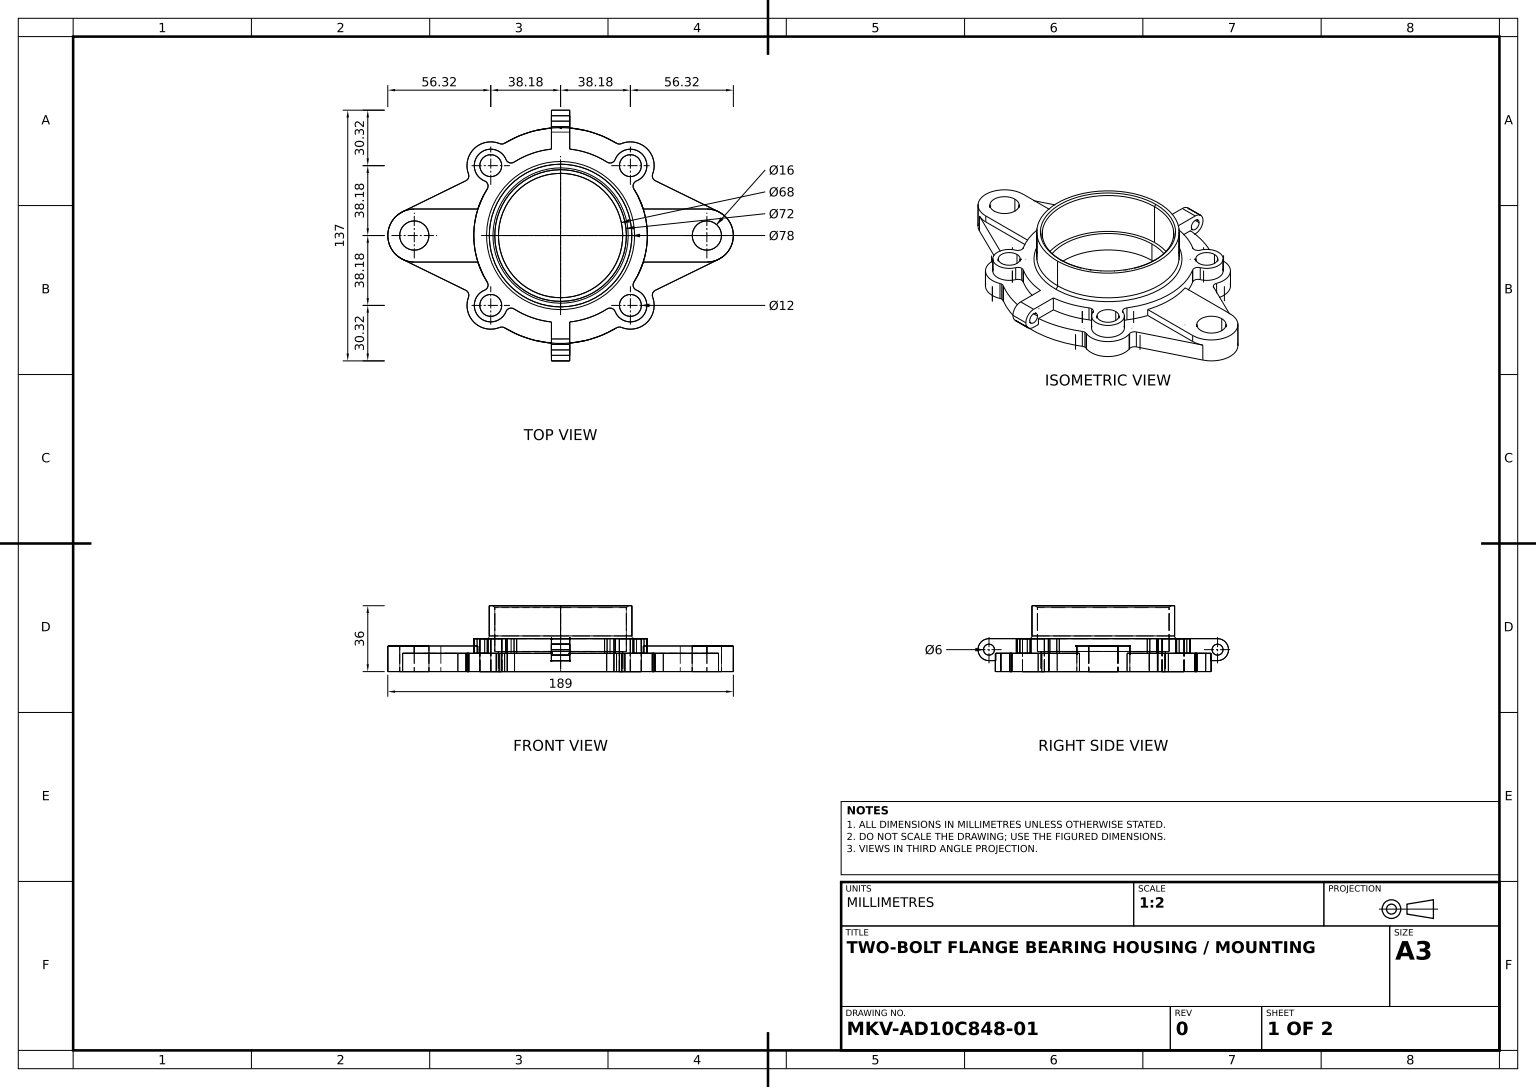
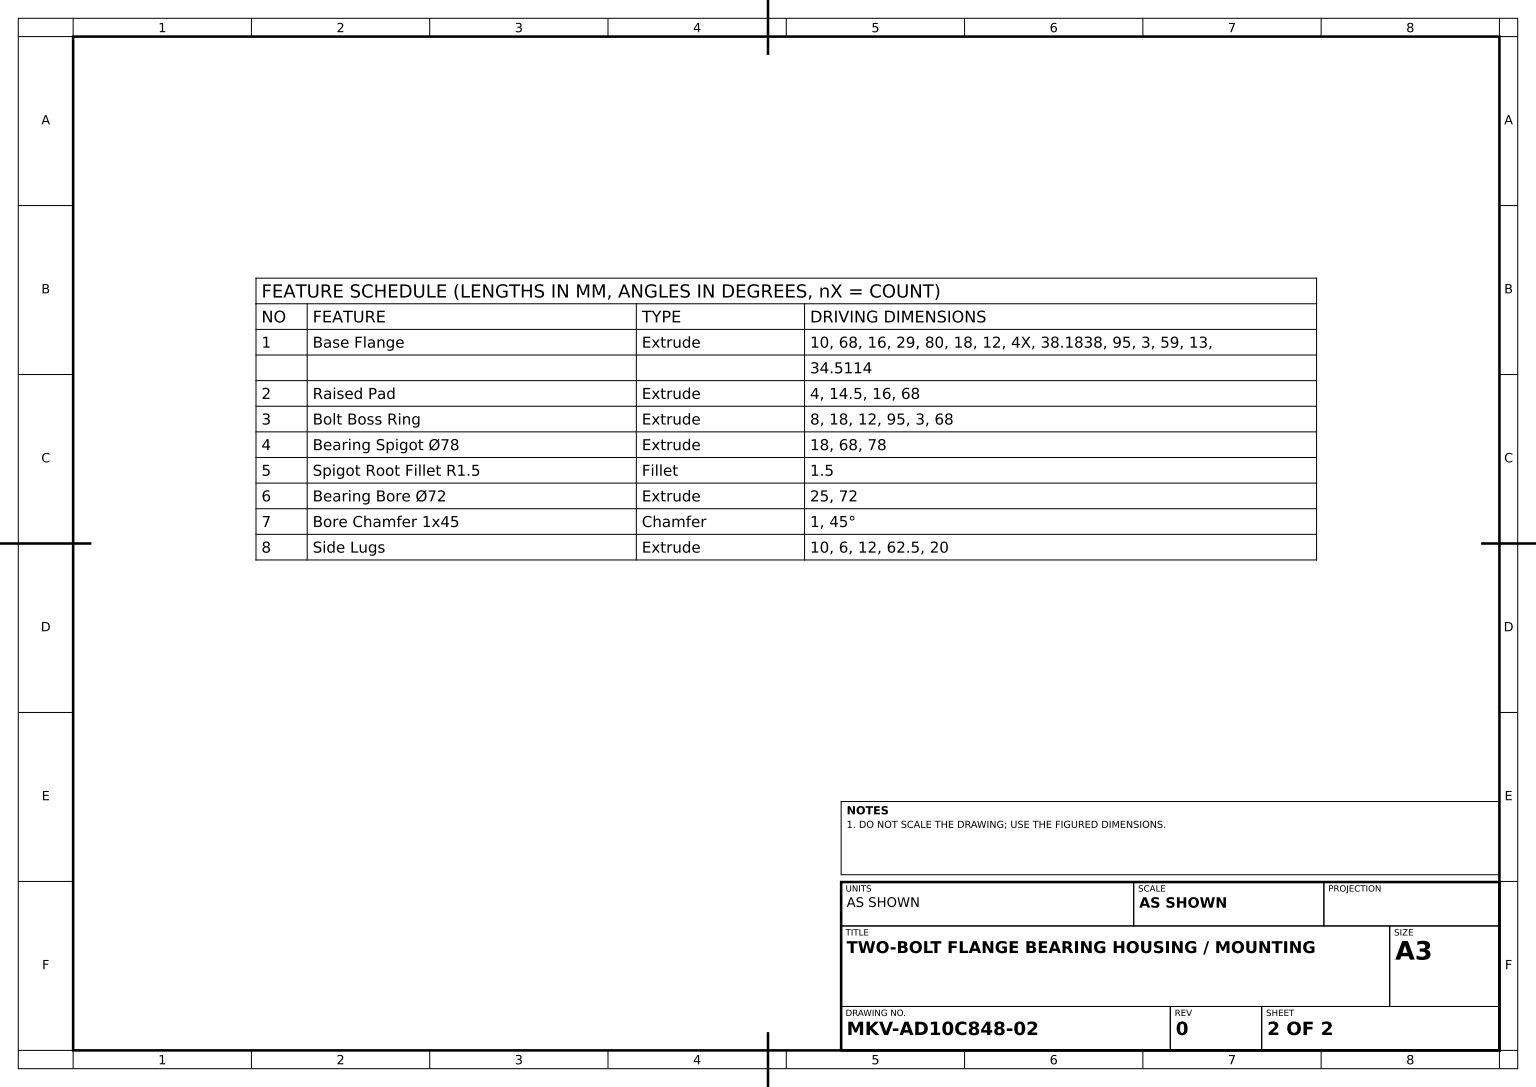
solid
v1 (5,10,47.236109)
v2 (25.438297,10,40.114125)
e1 v1 v2 CIRCLE(AX(P(0,10,0),D(0,1,0),D(0,0,1)),47.5)
v3 (25.438297,18,40.114125)
e2 v3 v2 LINE
v4 (5,18,47.236109)
e3 v4 v3 CIRCLE(AX(P(0,18,0),D(0,1,0),D(0,0,1)),47.5)
e4 v4 v1 LINE
face CYL(AX(P(0,18,0),D(0,-1,0),D(0,0,-1)),47.5) [e1 -e2 -e3 e4]
v5 (-30.604247,0,-50.441848)
v6 (-33.289778,0,-50.22739)
e5 v5 v6 CIRCLE(AX(P(-32.160396,0,-53.006688),D(0,-1,0),D(0,0,1)),3)
v7 (-33.289778,10,-50.22739)
e6 v7 v6 LINE
v8 (-30.604247,10,-50.441848)
e7 v8 v7 CIRCLE(AX(P(-32.160396,10,-53.006688),D(0,-1,0),D(0,0,1)),3)
e8 v8 v5 LINE
face CYL(AX(P(-32.160396,10,-53.006688),D(0,-1,0),D(0,0,-1)),3) rev [e5 -e6 -e7 e8]
v9 (38.183766,18,44.183766)
v10 (38.183766,18,32.183766)
e9 v9 v10 CIRCLE(AX(P(38.183766,18,38.183766),D(0,1,0),D(0,0,1)),6)
v11 (38.183766,0,32.183766)
e10 v10 v11 LINE
v12 (38.183766,0,44.183766)
e11 v12 v11 CIRCLE(AX(P(38.183766,0,38.183766),D(0,1,0),D(0,0,1)),6)
e12 v9 v12 LINE
face CYL(AX(P(38.183766,10,38.183766),D(0,-1,0),D(0,0,-1)),6) rev [e9 e10 -e11 -e12]
v13 (80,14,8)
v14 (80,0,8)
e13 v13 v14 LINE
v15 (80,14,-8)
e14 v13 v15 CIRCLE(AX(P(80,14,0),D(0,1,0),D(0,0,1)),8)
v16 (80,0,-8)
e15 v15 v16 LINE
e16 v14 v16 CIRCLE(AX(P(80,0,0),D(0,1,0),D(0,0,1)),8)
face CYL(AX(P(80,10,0),D(0,-1,0),D(0,0,-1)),8) rev [-e13 e14 e15 -e16]
v17 (27.044926,10,39.647649)
e17 v2 v17 CIRCLE(AX(P(27.044926,10,42.647649),D(0,-1,0),D(0,0,1)),3)
v18 (27.044926,18,39.647649)
e18 v18 v17 LINE
e19 v3 v18 CIRCLE(AX(P(27.044926,18,42.647649),D(0,-1,0),D(0,0,1)),3)
face CYL(AX(P(27.044926,18,42.647649),D(0,-1,0),D(0,0,-1)),3) rev [e17 -e18 -e19 e2]
v19 (29.829636,18,41.531678)
v20 (29.829636,10,41.531678)
e20 v19 v20 LINE
e21 v18 v19 CIRCLE(AX(P(27.044926,18,42.647649),D(0,-1,0),D(0,0,1)),3)
e22 v17 v20 CIRCLE(AX(P(27.044926,10,42.647649),D(0,-1,0),D(0,0,1)),3)
face CYL(AX(P(27.044926,18,42.647649),D(0,-1,0),D(0,0,-1)),3) rev [-e20 -e21 e18 e22]
v21 (-41.531678,18,-29.829636)
v22 (-41.531678,10,-29.829636)
e23 v21 v22 LINE
v23 (-38.183766,18,-47.183766)
e24 v23 v21 CIRCLE(AX(P(-38.183766,18,-38.183766),D(0,1,0),D(0,0,1)),9)
v24 (-38.183766,10,-47.183766)
e25 v23 v24 LINE
e26 v24 v22 CIRCLE(AX(P(-38.183766,10,-38.183766),D(0,1,0),D(0,0,1)),9)
face CYL(AX(P(-38.183766,18,-38.183766),D(0,-1,0),D(0,0,-1)),9) [-e23 -e24 e25 e26]
v25 (5,6,-62.5)
v26 (-5,6,-62.5)
e27 v25 v26 LINE
v27 (5,6,-58.787754)
e28 v27 v25 LINE
v28 (0,6,-59)
e29 v27 v28 CIRCLE(AX(P(0,6,0),D(0,1,0),D(0,0,1)),59)
v29 (-5,6,-58.787754)
e30 v28 v29 CIRCLE(AX(P(0,6,0),D(0,1,0),D(0,0,1)),59)
e31 v29 v26 LINE
face PLANE(AX(P(5,6,-42.5),D(0,1,0),D(0,0,1))) rev [-e27 -e28 e29 e30 e31]
v30 (32.160396,0,50.006688)
v31 (30.604247,0,50.441848)
e32 v30 v31 CIRCLE(AX(P(32.160396,0,53.006688),D(0,1,0),D(0,0,1)),3)
v32 (32.160396,10,50.006688)
e33 v32 v30 LINE
v33 (30.604247,10,50.441848)
e34 v32 v33 CIRCLE(AX(P(32.160396,10,53.006688),D(0,1,0),D(0,0,1)),3)
e35 v33 v31 LINE
face CYL(AX(P(32.160396,10,53.006688),D(0,-1,0),D(0,0,-1)),3) rev [-e32 -e33 e34 e35]
v34 (-50.367829,10,-33.650707)
v35 (-50.367829,0,-33.650707)
e36 v34 v35 LINE
v36 (-51.861087,0,-29.909864)
e37 v36 v35 CIRCLE(AX(P(-53.179535,0,-32.604617),D(0,1,0),D(0,0,1)),3)
v37 (-51.861087,10,-29.909864)
e38 v37 v36 LINE
e39 v37 v34 CIRCLE(AX(P(-53.179535,10,-32.604617),D(0,1,0),D(0,0,1)),3)
face CYL(AX(P(-53.179535,10,-32.604617),D(0,-1,0),D(0,0,-1)),3) rev [e36 -e37 -e38 e39]
v38 (-86.3725,10,-13.02464)
v39 (-86.3725,0,-13.02464)
e40 v38 v39 LINE
e41 v38 v37 LINE
e42 v39 v36 LINE
face PLANE(AX(P(-21.824105,10,-44.605905),D(-0.439482725,0,-0.898251042),D(-0.898251042,0,0.439482725))) [-e40 e41 e38 -e42]
v40 (0,11,-34)
v41 (0,11,34)
e43 v40 v41 CIRCLE(AX(P(0,11,0),D(0,1,0),D(0,0,1)),34)
v42 (0,0,34)
e44 v41 v42 LINE
v43 (0,0,-34)
e45 v43 v42 CIRCLE(AX(P(0,0,0),D(0,1,0),D(0,0,1)),34)
e46 v40 v43 LINE
face CYL(AX(P(0,10,0),D(0,-1,0),D(0,0,-1)),34) rev [e43 e44 -e45 -e46]
v44 (45.232732,14,-14.5)
v45 (45.232732,14,14.5)
e47 v44 v45 CIRCLE(AX(P(0,14,0),D(0,-1,0),D(0,0,1)),47.5)
v46 (45.232732,10,-14.5)
e48 v44 v46 LINE
v47 (40.114125,10,-25.438297)
e49 v46 v47 CIRCLE(AX(P(0,10,0),D(0,1,0),D(0,0,1)),47.5)
v48 (40.114125,18,-25.438297)
e50 v48 v47 LINE
v49 (40.114125,18,25.438297)
e51 v49 v48 CIRCLE(AX(P(0,18,0),D(0,1,0),D(0,0,1)),47.5)
v50 (40.114125,10,25.438297)
e52 v49 v50 LINE
v51 (45.232732,10,14.5)
e53 v50 v51 CIRCLE(AX(P(0,10,0),D(0,1,0),D(0,0,1)),47.5)
e54 v51 v45 LINE
face CYL(AX(P(0,18,0),D(0,-1,0),D(0,0,-1)),47.5) [-e47 e48 e49 -e50 -e51 e52 e53 e54]
v52 (38.183766,10,-51.183766)
v53 (33.289778,10,-50.22739)
e55 v52 v53 CIRCLE(AX(P(38.183766,10,-38.183766),D(0,1,0),D(0,0,1)),13)
v54 (38.183766,0,-51.183766)
e56 v52 v54 LINE
v55 (33.289778,0,-50.22739)
e57 v54 v55 CIRCLE(AX(P(38.183766,0,-38.183766),D(0,1,0),D(0,0,1)),13)
e58 v53 v55 LINE
face CYL(AX(P(38.183766,10,-38.183766),D(0,-1,0),D(0,0,-1)),13) [-e55 e56 e57 -e58]
v56 (30.604247,0,-50.441848)
e59 v55 v56 CIRCLE(AX(P(32.160396,0,-53.006688),D(0,-1,0),D(0,0,1)),3)
v57 (30.604247,10,-50.441848)
e60 v57 v56 LINE
e61 v53 v57 CIRCLE(AX(P(32.160396,10,-53.006688),D(0,-1,0),D(0,0,1)),3)
face CYL(AX(P(32.160396,10,-53.006688),D(0,-1,0),D(0,0,-1)),3) rev [e59 -e60 -e61 e58]
v58 (-80,14,14.5)
v59 (-80,10,14.5)
e62 v58 v59 LINE
v60 (-80,14,-14.5)
e63 v60 v58 CIRCLE(AX(P(-80,14,0),D(0,1,0),D(0,0,1)),14.5)
v61 (-80,10,-14.5)
e64 v60 v61 LINE
e65 v61 v38 CIRCLE(AX(P(-80,10,0),D(0,1,0),D(0,0,1)),14.5)
v62 (-86.3725,0,13.02464)
e66 v39 v62 CIRCLE(AX(P(-80,0,0),D(0,1,0),D(0,0,1)),14.5)
v63 (-86.3725,10,13.02464)
e67 v63 v62 LINE
e68 v59 v63 CIRCLE(AX(P(-80,10,0),D(0,-1,0),D(0,0,1)),14.5)
face CYL(AX(P(-80,10,0),D(0,-1,0),D(0,0,-1)),14.5) [-e62 -e63 e64 e65 e40 e66 -e67 -e68]
v64 (50.367829,10,33.650707)
v65 (50.367829,0,33.650707)
e69 v64 v65 LINE
v66 (51.861087,0,29.909864)
e70 v65 v66 CIRCLE(AX(P(53.179535,0,32.604617),D(0,-1,0),D(0,0,1)),3)
v67 (51.861087,10,29.909864)
e71 v67 v66 LINE
e72 v64 v67 CIRCLE(AX(P(53.179535,10,32.604617),D(0,-1,0),D(0,0,1)),3)
face CYL(AX(P(53.179535,10,32.604617),D(0,-1,0),D(0,0,-1)),3) rev [e69 e70 -e71 -e72]
v68 (-80,14,-8)
v69 (-80,14,8)
e73 v68 v69 CIRCLE(AX(P(-80,14,0),D(0,1,0),D(0,0,1)),8)
v70 (-80,0,8)
e74 v69 v70 LINE
v71 (-80,0,-8)
e75 v71 v70 CIRCLE(AX(P(-80,0,0),D(0,1,0),D(0,0,1)),8)
e76 v68 v71 LINE
face CYL(AX(P(-80,10,0),D(0,-1,0),D(0,0,-1)),8) rev [e73 e74 -e75 -e76]
v72 (-5,6,58.787754)
v73 (5,6,58.787754)
e77 v72 v73 CIRCLE(AX(P(0,6,0),D(0,1,0),D(0,0,1)),59)
v74 (5,6,62.5)
e78 v74 v73 LINE
v75 (-5,6,62.5)
e79 v74 v75 LINE
e80 v75 v72 LINE
face PLANE(AX(P(5,6,42.5),D(0,1,0),D(0,0,1))) rev [e77 -e78 e79 e80]
v76 (0,11,36)
v77 (0,35,36)
e81 v76 v77 LINE
v78 (0,35,-36)
e82 v77 v78 CIRCLE(AX(P(0,35,0),D(0,1,0),D(0,0,1)),36)
v79 (0,11,-36)
e83 v79 v78 LINE
e84 v76 v79 CIRCLE(AX(P(0,11,0),D(0,1,0),D(0,0,1)),36)
face CYL(AX(P(0,11,0),D(0,1,0),D(0,0,1)),36) rev [e81 e82 -e83 -e84]
v80 (80,10,14.5)
e85 v51 v80 LINE
v81 (80,14,14.5)
e86 v81 v80 LINE
e87 v45 v81 LINE
face PLANE(AX(P(80,14,14.5),D(0,0,-1),D(-1,0,0))) rev [e85 -e86 -e87 -e54]
v82 (-45.232732,14,-14.5)
e88 v82 v60 LINE
v83 (-45.232732,10,-14.5)
e89 v83 v82 LINE
e90 v83 v61 LINE
face PLANE(AX(P(-80,14,-14.5),D(0,0,1),D(1,0,0))) rev [-e64 -e88 -e89 e90]
v84 (-40.114125,10,25.438297)
v85 (-41.531678,10,29.829636)
e91 v84 v85 CIRCLE(AX(P(-42.647649,10,27.044926),D(0,-1,0),D(0,0,1)),3)
v86 (-45.232732,10,14.5)
e92 v86 v84 CIRCLE(AX(P(0,10,0),D(0,1,0),D(0,0,1)),47.5)
e93 v59 v86 LINE
v87 (-51.861087,10,29.909864)
e94 v63 v87 LINE
v88 (-50.367829,10,33.650707)
e95 v87 v88 CIRCLE(AX(P(-53.179535,10,32.604617),D(0,-1,0),D(0,0,1)),3)
v89 (-33.289778,10,50.22739)
e96 v88 v89 CIRCLE(AX(P(-38.183766,10,38.183766),D(0,1,0),D(0,0,1)),13)
v90 (-32.160396,10,50.006688)
e97 v90 v89 CIRCLE(AX(P(-32.160396,10,53.006688),D(0,1,0),D(0,0,1)),3)
v91 (-30.604247,10,50.441848)
e98 v91 v90 CIRCLE(AX(P(-32.160396,10,53.006688),D(0,1,0),D(0,0,1)),3)
v92 (-5,10,58.787754)
e99 v91 v92 CIRCLE(AX(P(0,10,0),D(0,1,0),D(0,0,1)),59)
v93 (-5,10,47.236109)
e100 v92 v93 LINE
v94 (-25.438297,10,40.114125)
e101 v94 v93 CIRCLE(AX(P(0,10,0),D(0,1,0),D(0,0,1)),47.5)
v95 (-27.044926,10,39.647649)
e102 v95 v94 CIRCLE(AX(P(-27.044926,10,42.647649),D(0,-1,0),D(0,0,-1)),3)
v96 (-29.829636,10,41.531678)
e103 v96 v95 CIRCLE(AX(P(-27.044926,10,42.647649),D(0,-1,0),D(0,0,-1)),3)
e104 v85 v96 CIRCLE(AX(P(-38.183766,10,38.183766),D(0,1,0),D(0,0,1)),9)
face PLANE(AX(P(0,10,0),D(0,1,0),D(0,0,1))) [-e91 -e92 -e93 e68 e94 e95 e96 -e97 -e98 e99 e100 -e101 -e102 -e103 -e104]
v97 (-25.438297,10,-40.114125)
v98 (-29.829636,10,-41.531678)
e105 v97 v98 CIRCLE(AX(P(-27.044926,10,-42.647649),D(0,-1,0),D(0,0,1)),3)
v99 (-29.829636,18,-41.531678)
e106 v99 v98 LINE
v100 (-25.438297,18,-40.114125)
e107 v100 v99 CIRCLE(AX(P(-27.044926,18,-42.647649),D(0,-1,0),D(0,0,1)),3)
e108 v100 v97 LINE
face CYL(AX(P(-27.044926,18,-42.647649),D(0,-1,0),D(0,0,-1)),3) rev [e105 -e106 -e107 e108]
v101 (25.438297,18,-40.114125)
v102 (25.438297,10,-40.114125)
e109 v101 v102 LINE
v103 (5,10,-47.236109)
e110 v102 v103 CIRCLE(AX(P(0,10,0),D(0,1,0),D(0,0,1)),47.5)
v104 (5,18,-47.236109)
e111 v103 v104 LINE
e112 v101 v104 CIRCLE(AX(P(0,18,0),D(0,1,0),D(0,0,1)),47.5)
face CYL(AX(P(0,18,0),D(0,-1,0),D(0,0,-1)),47.5) [e109 e110 e111 -e112]
v105 (51.861087,10,-29.909864)
v106 (50.367829,10,-33.650707)
e113 v105 v106 CIRCLE(AX(P(53.179535,10,-32.604617),D(0,-1,0),D(0,0,1)),3)
v107 (51.861087,0,-29.909864)
e114 v105 v107 LINE
v108 (50.367829,0,-33.650707)
e115 v107 v108 CIRCLE(AX(P(53.179535,0,-32.604617),D(0,-1,0),D(0,0,1)),3)
e116 v106 v108 LINE
face CYL(AX(P(53.179535,10,-32.604617),D(0,-1,0),D(0,0,-1)),3) rev [-e113 e114 e115 -e116]
v109 (0,18,40.5)
v110 (0,19.5,39)
e117 v109 v110 CIRCLE(AX(P(0,19.5,40.5),D(1,0,0),D(0,0,-1)),1.5)
v111 (0,18,-40.5)
e118 v111 v109 CIRCLE(AX(P(0,18,0),D(0,-1,0),D(0,0,-1)),40.5)
v112 (0,19.5,-39)
e119 v111 v112 CIRCLE(AX(P(0,19.5,-40.5),D(-1,0,0),D(0,0,1)),1.5)
e120 v110 v112 CIRCLE(AX(P(0,19.5,0),D(0,1,0),D(0,0,-1)),39)
face TORUS(AX(P(0,19.5,0),D(0,-1,0),D(0,0,-1)),40.5,1.5) rev [-e117 -e118 e119 -e120]
v113 (41.531678,18,-29.829636)
e121 v48 v113 CIRCLE(AX(P(42.647649,18,-27.044926),D(0,-1,0),D(0,0,1)),3)
v114 (41.531678,10,-29.829636)
e122 v47 v114 CIRCLE(AX(P(42.647649,10,-27.044926),D(0,-1,0),D(0,0,1)),3)
e123 v113 v114 LINE
face CYL(AX(P(42.647649,18,-27.044926),D(0,-1,0),D(0,0,-1)),3) rev [-e121 e50 e122 -e123]
v115 (-5,18,-47.236109)
e124 v115 v100 CIRCLE(AX(P(0,18,0),D(0,1,0),D(0,0,1)),47.5)
v116 (-5,10,-47.236109)
e125 v116 v115 LINE
e126 v116 v97 CIRCLE(AX(P(0,10,0),D(0,1,0),D(0,0,1)),47.5)
face CYL(AX(P(0,18,0),D(0,-1,0),D(0,0,-1)),47.5) [-e124 -e125 e126 -e108]
v117 (5,12,-59.5)
v118 (5,12,-65.5)
e127 v117 v118 CIRCLE(AX(P(5,12,-62.5),D(1,0,0),D(0,0,-1)),3)
e128 v118 v117 CIRCLE(AX(P(5,12,-62.5),D(1,0,0),D(0,0,-1)),3)
v119 (5,10,-58.787754)
e129 v27 v119 LINE
v120 (5,18,-62.5)
e130 v25 v120 CIRCLE(AX(P(5,12,-62.5),D(1,0,0),D(0,0,-1)),6)
e131 v120 v104 LINE
e132 v103 v119 LINE
face PLANE(AX(P(5,12,-62.5),D(1,0,0),D(0,0,-1))) [-e127 -e128] [-e129 e28 e130 e131 -e111 e132]
v121 (-5,12,-59.5)
e133 v117 v121 LINE
v122 (-5,12,-65.5)
e134 v122 v121 CIRCLE(AX(P(-5,12,-62.5),D(1,0,0),D(0,0,-1)),3)
e135 v118 v122 LINE
face CYL(AX(P(5,12,-62.5),D(-1,0,0),D(0,0,1)),3) rev [e128 e133 -e134 -e135]
v123 (-5,18,62.5)
v124 (-5,12,68.5)
e136 v123 v124 CIRCLE(AX(P(-5,12,62.5),D(1,0,0),D(0,0,-1)),6)
v125 (5,12,68.5)
e137 v125 v124 LINE
v126 (5,18,62.5)
e138 v126 v125 CIRCLE(AX(P(5,12,62.5),D(1,0,0),D(0,0,-1)),6)
e139 v126 v123 LINE
face CYL(AX(P(5,12,62.5),D(-1,0,0),D(0,0,1)),6) [e136 -e137 -e138 e139]
v127 (86.3725,10,13.02464)
v128 (86.3725,0,13.02464)
e140 v127 v128 LINE
v129 (86.3725,0,-13.02464)
e141 v128 v129 CIRCLE(AX(P(80,0,0),D(0,1,0),D(0,0,1)),14.5)
v130 (86.3725,10,-13.02464)
e142 v130 v129 LINE
v131 (80,10,-14.5)
e143 v130 v131 CIRCLE(AX(P(80,10,0),D(0,1,0),D(0,0,1)),14.5)
v132 (80,14,-14.5)
e144 v132 v131 LINE
e145 v81 v132 CIRCLE(AX(P(80,14,0),D(0,1,0),D(0,0,1)),14.5)
e146 v80 v127 CIRCLE(AX(P(80,10,0),D(0,1,0),D(0,0,1)),14.5)
face CYL(AX(P(80,10,0),D(0,-1,0),D(0,0,-1)),14.5) [e140 e141 -e142 e143 -e144 -e145 e86 e146]
v133 (-27.044926,18,39.647649)
e147 v133 v95 LINE
v134 (-25.438297,18,40.114125)
e148 v134 v94 LINE
e149 v133 v134 CIRCLE(AX(P(-27.044926,18,42.647649),D(0,-1,0),D(0,0,-1)),3)
face CYL(AX(P(-27.044926,18,42.647649),D(0,-1,0),D(0,0,-1)),3) rev [e147 e102 -e148 -e149]
v135 (-38.183766,0,44.183766)
v136 (-38.183766,0,32.183766)
e150 v135 v136 CIRCLE(AX(P(-38.183766,0,38.183766),D(0,1,0),D(0,0,1)),6)
v137 (-38.183766,18,44.183766)
e151 v137 v135 LINE
v138 (-38.183766,18,32.183766)
e152 v137 v138 CIRCLE(AX(P(-38.183766,18,38.183766),D(0,1,0),D(0,0,1)),6)
e153 v138 v136 LINE
face CYL(AX(P(-38.183766,10,38.183766),D(0,-1,0),D(0,0,-1)),6) rev [-e150 -e151 e152 e153]
v139 (-51.861087,0,29.909864)
e154 v62 v139 LINE
e155 v87 v139 LINE
face PLANE(AX(P(-21.824105,10,44.605905),D(0.439482725,0,-0.898251042),D(-0.898251042,0,-0.439482725))) rev [e67 e154 -e155 -e94]
v140 (-30.604247,0,50.441848)
e156 v91 v140 LINE
v141 (-32.160396,0,50.006688)
e157 v90 v141 LINE
e158 v140 v141 CIRCLE(AX(P(-32.160396,0,53.006688),D(0,1,0),D(0,0,1)),3)
face CYL(AX(P(-32.160396,10,53.006688),D(0,-1,0),D(0,0,-1)),3) rev [-e156 e98 e157 -e158]
v142 (33.289778,10,50.22739)
e159 v142 v64 CIRCLE(AX(P(38.183766,10,38.183766),D(0,1,0),D(0,0,1)),13)
v143 (33.289778,0,50.22739)
e160 v142 v143 LINE
e161 v143 v65 CIRCLE(AX(P(38.183766,0,38.183766),D(0,1,0),D(0,0,1)),13)
face CYL(AX(P(38.183766,10,38.183766),D(0,-1,0),D(0,0,-1)),13) [-e69 -e159 e160 e161]
e162 v127 v67 LINE
e163 v128 v66 LINE
face PLANE(AX(P(21.824105,10,44.605905),D(0.439482725,0,0.898251042),D(0.898251042,0,-0.439482725))) [e162 e71 -e163 -e140]
v144 (41.531678,18,29.829636)
v145 (41.531678,10,29.829636)
e164 v144 v145 LINE
e165 v19 v144 CIRCLE(AX(P(38.183766,18,38.183766),D(0,1,0),D(0,0,1)),9)
e166 v20 v145 CIRCLE(AX(P(38.183766,10,38.183766),D(0,1,0),D(0,0,1)),9)
face CYL(AX(P(38.183766,18,38.183766),D(0,-1,0),D(0,0,-1)),9) [-e164 -e165 e20 e166]
v146 (-45.232732,14,14.5)
e167 v146 v86 LINE
e168 v58 v146 LINE
face PLANE(AX(P(-30.753049,14,14.5),D(0,0,-1),D(-1,0,0))) rev [e93 -e167 -e168 e62]
e169 v69 v68 CIRCLE(AX(P(-80,14,0),D(0,1,0),D(0,0,1)),8)
e170 v146 v82 CIRCLE(AX(P(0,14,0),D(0,-1,0),D(0,0,1)),47.5)
face PLANE(AX(P(0,14,0),D(0,1,0),D(0,0,1))) [-e73 -e169] [e88 e63 e168 e170]
v147 (-38.183766,18,-44.183766)
v148 (-38.183766,0,-44.183766)
e171 v147 v148 LINE
v149 (-38.183766,0,-32.183766)
e172 v149 v148 CIRCLE(AX(P(-38.183766,0,-38.183766),D(0,1,0),D(0,0,1)),6)
v150 (-38.183766,18,-32.183766)
e173 v150 v149 LINE
e174 v150 v147 CIRCLE(AX(P(-38.183766,18,-38.183766),D(0,1,0),D(0,0,1)),6)
face CYL(AX(P(-38.183766,10,-38.183766),D(0,-1,0),D(0,0,-1)),6) rev [e171 -e172 -e173 e174]
v151 (-50.367829,0,33.650707)
e175 v88 v151 LINE
e176 v139 v151 CIRCLE(AX(P(-53.179535,0,32.604617),D(0,-1,0),D(0,0,1)),3)
face CYL(AX(P(-53.179535,10,32.604617),D(0,-1,0),D(0,0,-1)),3) rev [-e175 -e95 e155 e176]
e177 v125 v74 CIRCLE(AX(P(5,12,62.5),D(1,0,0),D(0,0,-1)),6)
v152 (5,10,58.787754)
e178 v152 v73 LINE
e179 v152 v1 LINE
e180 v4 v126 LINE
v153 (5,12,65.5)
v154 (5,12,59.5)
e181 v153 v154 CIRCLE(AX(P(5,12,62.5),D(1,0,0),D(0,0,-1)),3)
e182 v154 v153 CIRCLE(AX(P(5,12,62.5),D(1,0,0),D(0,0,-1)),3)
face PLANE(AX(P(5,12,62.5),D(1,0,0),D(0,0,-1))) [e138 e177 e78 -e178 e179 -e4 e180] [-e181 -e182]
e183 v70 v71 CIRCLE(AX(P(-80,0,0),D(0,1,0),D(0,0,1)),8)
face CYL(AX(P(-80,10,0),D(0,-1,0),D(0,0,-1)),8) rev [-e74 e169 e76 -e183]
v155 (-5,12,65.5)
e184 v153 v155 LINE
v156 (-5,12,59.5)
e185 v156 v155 CIRCLE(AX(P(-5,12,62.5),D(1,0,0),D(0,0,-1)),3)
e186 v154 v156 LINE
face CYL(AX(P(5,12,62.5),D(-1,0,0),D(0,0,1)),3) rev [e182 e184 -e185 -e186]
e187 v57 v119 CIRCLE(AX(P(0,10,0),D(0,1,0),D(0,0,1)),59)
v157 (0,0,-59)
e188 v56 v157 CIRCLE(AX(P(0,0,0),D(0,1,0),D(0,0,1)),59)
e189 v28 v157 LINE
face CYL(AX(P(0,10,0),D(0,-1,0),D(0,0,-1)),59) [-e187 e60 e188 -e189 -e29 e129]
e190 v15 v13 CIRCLE(AX(P(80,14,0),D(0,1,0),D(0,0,1)),8)
e191 v16 v14 CIRCLE(AX(P(80,0,0),D(0,1,0),D(0,0,1)),8)
face CYL(AX(P(80,10,0),D(0,-1,0),D(0,0,-1)),8) rev [-e15 e190 e13 -e191]
e192 v143 v30 CIRCLE(AX(P(32.160396,0,53.006688),D(0,1,0),D(0,0,1)),3)
e193 v142 v32 CIRCLE(AX(P(32.160396,10,53.006688),D(0,1,0),D(0,0,1)),3)
face CYL(AX(P(32.160396,10,53.006688),D(0,-1,0),D(0,0,-1)),3) rev [e33 -e192 -e160 e193]
e194 v121 v122 CIRCLE(AX(P(-5,12,-62.5),D(1,0,0),D(0,0,-1)),3)
face CYL(AX(P(5,12,-62.5),D(-1,0,0),D(0,0,1)),3) rev [e127 e135 -e194 -e133]
v158 (0,36,39)
v159 (0,36,-39)
e195 v158 v159 CIRCLE(AX(P(0,36,0),D(0,1,0),D(0,0,1)),39)
e196 v158 v110 LINE
e197 v159 v112 LINE
face CYL(AX(P(0,36,0),D(0,-1,0),D(0,0,-1)),39) [-e195 e196 e120 -e197]
v160 (-5,18,47.236109)
e198 v160 v93 LINE
e199 v134 v160 CIRCLE(AX(P(0,18,0),D(0,1,0),D(0,0,1)),47.5)
face CYL(AX(P(0,18,0),D(0,-1,0),D(0,0,-1)),47.5) [e101 -e198 -e199 e148]
v161 (-5,10,-58.787754)
e200 v116 v161 LINE
e201 v161 v8 CIRCLE(AX(P(0,10,0),D(0,1,0),D(0,0,1)),59)
v162 (-38.183766,10,-51.183766)
e202 v7 v162 CIRCLE(AX(P(-38.183766,10,-38.183766),D(0,1,0),D(0,0,1)),13)
e203 v162 v34 CIRCLE(AX(P(-38.183766,10,-38.183766),D(0,1,0),D(0,0,1)),13)
v163 (-40.114125,10,-25.438297)
e204 v163 v83 CIRCLE(AX(P(0,10,0),D(0,1,0),D(0,0,1)),47.5)
e205 v22 v163 CIRCLE(AX(P(-42.647649,10,-27.044926),D(0,-1,0),D(0,0,-1)),3)
e206 v98 v24 CIRCLE(AX(P(-38.183766,10,-38.183766),D(0,1,0),D(0,0,1)),9)
face PLANE(AX(P(0,10,0),D(0,1,0),D(0,0,1))) [-e105 -e126 e200 e201 e7 e202 e203 -e39 -e41 -e65 -e90 -e204 -e205 -e26 -e206]
e207 v11 v12 CIRCLE(AX(P(38.183766,0,38.183766),D(0,1,0),D(0,0,1)),6)
e208 v10 v9 CIRCLE(AX(P(38.183766,18,38.183766),D(0,1,0),D(0,0,1)),6)
face CYL(AX(P(38.183766,10,38.183766),D(0,-1,0),D(0,0,-1)),6) rev [-e207 -e10 e208 e12]
e209 v41 v40 CIRCLE(AX(P(0,11,0),D(0,1,0),D(0,0,1)),34)
e210 v79 v76 CIRCLE(AX(P(0,11,0),D(0,1,0),D(0,0,1)),36)
face PLANE(AX(P(0,11,0),D(0,1,0),D(0,0,1))) [-e43 -e209] [e210 e84]
v164 (-33.289778,0,50.22739)
e211 v89 v164 LINE
e212 v141 v164 CIRCLE(AX(P(-32.160396,0,53.006688),D(0,1,0),D(0,0,1)),3)
face CYL(AX(P(-32.160396,10,53.006688),D(0,-1,0),D(0,0,-1)),3) rev [-e157 e97 e211 -e212]
e213 v144 v49 CIRCLE(AX(P(42.647649,18,27.044926),D(0,-1,0),D(0,0,-1)),3)
e214 v145 v50 CIRCLE(AX(P(42.647649,10,27.044926),D(0,-1,0),D(0,0,-1)),3)
face CYL(AX(P(42.647649,18,27.044926),D(0,-1,0),D(0,0,-1)),3) rev [-e213 e164 e214 -e52]
e215 v42 v43 CIRCLE(AX(P(0,0,0),D(0,1,0),D(0,0,1)),34)
e216 v136 v135 CIRCLE(AX(P(-38.183766,0,38.183766),D(0,1,0),D(0,0,1)),6)
e217 v148 v149 CIRCLE(AX(P(-38.183766,0,-38.183766),D(0,1,0),D(0,0,1)),6)
v165 (38.183766,0,-44.183766)
v166 (38.183766,0,-32.183766)
e218 v165 v166 CIRCLE(AX(P(38.183766,0,-38.183766),D(0,1,0),D(0,0,1)),6)
e219 v166 v165 CIRCLE(AX(P(38.183766,0,-38.183766),D(0,1,0),D(0,0,1)),6)
v167 (-38.183766,0,-51.183766)
e220 v167 v35 CIRCLE(AX(P(-38.183766,0,-38.183766),D(0,1,0),D(0,0,1)),13)
e221 v6 v167 CIRCLE(AX(P(-38.183766,0,-38.183766),D(0,1,0),D(0,0,1)),13)
e222 v157 v5 CIRCLE(AX(P(0,0,0),D(0,1,0),D(0,0,1)),59)
e223 v108 v54 CIRCLE(AX(P(38.183766,0,-38.183766),D(0,1,0),D(0,0,1)),13)
e224 v129 v107 LINE
e225 v140 v31 CIRCLE(AX(P(0,0,0),D(0,1,0),D(0,0,1)),59)
e226 v151 v164 CIRCLE(AX(P(-38.183766,0,38.183766),D(0,1,0),D(0,0,1)),13)
face PLANE(AX(P(0,0,0),D(0,1,0),D(0,0,1))) rev [e45 e215] [e216 e150] [e217 e172] [e218 e219] [e191 e16] [e75 e183] [e207 e11] [-e154 -e66 e42 e37 -e220 -e221 -e5 -e222 -e188 -e59 -e57 -e223 -e115 -e224 -e141 e163 -e70 -e161 e192 e32 -e225 e158 e212 -e226 -e176]
v168 (-29.829636,18,41.531678)
e227 v168 v133 CIRCLE(AX(P(-27.044926,18,42.647649),D(0,-1,0),D(0,0,-1)),3)
e228 v168 v96 LINE
face CYL(AX(P(-27.044926,18,42.647649),D(0,-1,0),D(0,0,-1)),3) rev [-e227 e228 e103 -e147]
v169 (-41.531678,18,29.829636)
e229 v169 v168 CIRCLE(AX(P(-38.183766,18,38.183766),D(0,1,0),D(0,0,1)),9)
e230 v169 v85 LINE
face CYL(AX(P(-38.183766,18,38.183766),D(0,-1,0),D(0,0,-1)),9) [e104 -e228 -e229 e230]
v170 (0,36,37)
v171 (0,36,-37)
e231 v170 v171 CIRCLE(AX(P(0,36,0),D(0,-1,0),D(0,0,1)),37)
e232 v77 v170 LINE
e233 v78 v77 CIRCLE(AX(P(0,35,0),D(0,1,0),D(0,0,1)),36)
e234 v78 v171 LINE
face CONE(AX(P(0,35,0),D(0,1,0),D(0,0,1)),36,0.785398163) rev [-e231 -e232 -e233 e234]
e235 v152 v33 CIRCLE(AX(P(0,10,0),D(0,1,0),D(0,0,1)),59)
face PLANE(AX(P(0,10,0),D(0,1,0),D(0,0,1))) [e235 -e34 -e193 e159 e72 -e162 -e146 -e85 -e53 -e214 -e166 -e22 -e17 -e1 -e179]
e236 v109 v111 CIRCLE(AX(P(0,18,0),D(0,-1,0),D(0,0,-1)),40.5)
e237 v112 v110 CIRCLE(AX(P(0,19.5,0),D(0,1,0),D(0,0,-1)),39)
face TORUS(AX(P(0,19.5,0),D(0,-1,0),D(0,0,-1)),40.5,1.5) rev [-e119 -e236 e117 -e237]
e238 v132 v44 LINE
e239 v131 v46 LINE
face PLANE(AX(P(30.753049,14,-14.5),D(0,0,1),D(1,0,0))) rev [-e48 -e238 e144 e239]
e240 v124 v75 CIRCLE(AX(P(-5,12,62.5),D(1,0,0),D(0,0,-1)),6)
face CYL(AX(P(5,12,62.5),D(-1,0,0),D(0,0,1)),6) [-e177 e137 e240 -e79]
e241 v138 v137 CIRCLE(AX(P(-38.183766,18,38.183766),D(0,1,0),D(0,0,1)),6)
face CYL(AX(P(-38.183766,10,38.183766),D(0,-1,0),D(0,0,-1)),6) rev [e151 -e216 -e153 e241]
e242 v160 v123 LINE
e243 v92 v72 LINE
e244 v155 v156 CIRCLE(AX(P(-5,12,62.5),D(1,0,0),D(0,0,-1)),3)
face PLANE(AX(P(-5,12,62.5),D(1,0,0),D(0,0,-1))) rev [-e242 e198 -e100 e243 -e80 -e240 -e136] [e244 e185]
face CYL(AX(P(5,12,62.5),D(-1,0,0),D(0,0,1)),3) rev [-e244 -e184 e181 e186]
e245 v159 v158 CIRCLE(AX(P(0,36,0),D(0,1,0),D(0,0,1)),39)
e246 v171 v170 CIRCLE(AX(P(0,36,0),D(0,-1,0),D(0,0,1)),37)
face PLANE(AX(P(0,36,0),D(0,1,0),D(0,0,1))) [e195 e245] [e246 e231]
e247 v147 v150 CIRCLE(AX(P(-38.183766,18,-38.183766),D(0,1,0),D(0,0,1)),6)
face CYL(AX(P(-38.183766,10,-38.183766),D(0,-1,0),D(0,0,-1)),6) rev [-e171 e247 e173 -e217]
face CYL(AX(P(0,10,0),D(0,-1,0),D(0,0,-1)),59) [e156 e225 -e35 -e235 e178 -e77 -e243 -e99]
v172 (29.829636,18,-41.531678)
e248 v172 v101 CIRCLE(AX(P(27.044926,18,-42.647649),D(0,-1,0),D(0,0,-1)),3)
v173 (29.829636,10,-41.531678)
e249 v172 v173 LINE
e250 v173 v102 CIRCLE(AX(P(27.044926,10,-42.647649),D(0,-1,0),D(0,0,-1)),3)
face CYL(AX(P(27.044926,18,-42.647649),D(0,-1,0),D(0,0,-1)),3) rev [-e248 e249 e250 -e109]
v174 (38.183766,18,-32.183766)
v175 (38.183766,18,-44.183766)
e251 v174 v175 CIRCLE(AX(P(38.183766,18,-38.183766),D(0,1,0),D(0,0,1)),6)
e252 v175 v165 LINE
e253 v174 v166 LINE
face CYL(AX(P(38.183766,10,-38.183766),D(0,-1,0),D(0,0,-1)),6) rev [e251 e252 -e219 -e253]
e254 v175 v174 CIRCLE(AX(P(38.183766,18,-38.183766),D(0,1,0),D(0,0,1)),6)
v176 (38.183766,18,-47.183766)
e255 v113 v176 CIRCLE(AX(P(38.183766,18,-38.183766),D(0,1,0),D(0,0,1)),9)
e256 v176 v172 CIRCLE(AX(P(38.183766,18,-38.183766),D(0,1,0),D(0,0,1)),9)
v177 (-5,18,-62.5)
e257 v120 v177 LINE
e258 v177 v115 LINE
e259 v99 v23 CIRCLE(AX(P(-38.183766,18,-38.183766),D(0,1,0),D(0,0,1)),9)
v178 (-40.114125,18,-25.438297)
e260 v21 v178 CIRCLE(AX(P(-42.647649,18,-27.044926),D(0,-1,0),D(0,0,-1)),3)
v179 (-40.114125,18,25.438297)
e261 v178 v179 CIRCLE(AX(P(0,18,0),D(0,1,0),D(0,0,1)),47.5)
e262 v179 v169 CIRCLE(AX(P(-42.647649,18,27.044926),D(0,-1,0),D(0,0,1)),3)
face PLANE(AX(P(21.323824,18,13.522463),D(0,-1,0),D(0,0,-1))) rev [-e208 -e9] [-e152 -e241] [-e254 -e251] [e213 e51 e121 e255 e256 e248 e112 -e131 e257 e258 e124 e107 e259 e24 e260 e261 e262 e229 e227 e149 e199 e242 -e139 -e180 e3 e19 e21 e165] [e118 e236] [-e174 -e247]
face CYL(AX(P(-38.183766,18,-38.183766),D(0,-1,0),D(0,0,-1)),9) [-e259 e106 e206 -e25]
e263 v130 v105 LINE
face PLANE(AX(P(21.824105,10,-44.605905),D(-0.439482725,0,0.898251042),D(0.898251042,0,0.439482725))) rev [e224 -e114 -e263 e142]
v180 (38.183766,10,-47.183766)
e264 v114 v180 CIRCLE(AX(P(38.183766,10,-38.183766),D(0,1,0),D(0,0,1)),9)
e265 v176 v180 LINE
face CYL(AX(P(38.183766,18,-38.183766),D(0,-1,0),D(0,0,-1)),9) [e264 -e265 -e255 e123]
face PLANE(AX(P(0,14,0),D(0,1,0),D(0,0,1))) [-e190 -e14] [e87 e145 e238 e47]
e266 v180 v173 CIRCLE(AX(P(38.183766,10,-38.183766),D(0,1,0),D(0,0,1)),9)
face CYL(AX(P(38.183766,18,-38.183766),D(0,-1,0),D(0,0,-1)),9) [-e256 e265 e266 -e249]
e267 v179 v84 LINE
face CYL(AX(P(-42.647649,18,27.044926),D(0,-1,0),D(0,0,-1)),3) rev [-e230 -e262 e267 e91]
e268 v26 v177 CIRCLE(AX(P(-5,12,-62.5),D(1,0,0),D(0,0,-1)),6)
face CYL(AX(P(5,12,-62.5),D(-1,0,0),D(0,0,1)),6) [-e257 -e130 e27 e268]
face CYL(AX(P(0,36,0),D(0,-1,0),D(0,0,-1)),39) [e237 -e196 -e245 e197]
e269 v29 v161 LINE
face PLANE(AX(P(-5,12,-62.5),D(1,0,0),D(0,0,-1))) rev [-e268 -e31 e269 -e200 e125 -e258] [e194 e134]
e270 v178 v163 LINE
face CYL(AX(P(-42.647649,18,-27.044926),D(0,-1,0),D(0,0,-1)),3) rev [-e270 -e260 e23 e205]
e271 v162 v167 LINE
face CYL(AX(P(-38.183766,10,-38.183766),D(0,-1,0),D(0,0,-1)),13) [-e36 -e203 e271 e220]
face CYL(AX(P(-38.183766,10,-38.183766),D(0,-1,0),D(0,0,-1)),13) [e221 -e271 -e202 e6]
face CYL(AX(P(0,18,0),D(0,-1,0),D(0,0,-1)),47.5) [e167 e92 -e267 -e261 e270 e204 e89 -e170]
face CYL(AX(P(38.183766,10,-38.183766),D(0,-1,0),D(0,0,-1)),6) rev [e254 e253 -e218 -e252]
face CYL(AX(P(-38.183766,10,38.183766),D(0,-1,0),D(0,0,-1)),13) [-e96 e175 e226 -e211]
e272 v106 v52 CIRCLE(AX(P(38.183766,10,-38.183766),D(0,1,0),D(0,0,1)),13)
face PLANE(AX(P(0,10,0),D(0,1,0),D(0,0,1))) [-e132 -e110 -e250 -e266 -e264 -e122 -e49 -e239 -e143 e263 e113 e272 e55 e61 e187]
face CYL(AX(P(0,10,0),D(0,-1,0),D(0,0,-1)),59) [e189 e222 -e8 -e201 -e269 -e30]
face CYL(AX(P(38.183766,10,-38.183766),D(0,-1,0),D(0,0,-1)),13) [e116 e223 -e56 -e272]
face CONE(AX(P(0,35,0),D(0,1,0),D(0,0,1)),36,0.785398163) rev [-e234 -e82 e232 -e246]
face CYL(AX(P(0,11,0),D(0,1,0),D(0,0,1)),36) rev [e233 -e81 -e210 e83]
face CYL(AX(P(0,10,0),D(0,-1,0),D(0,0,-1)),34) rev [e209 e46 -e215 -e44]
